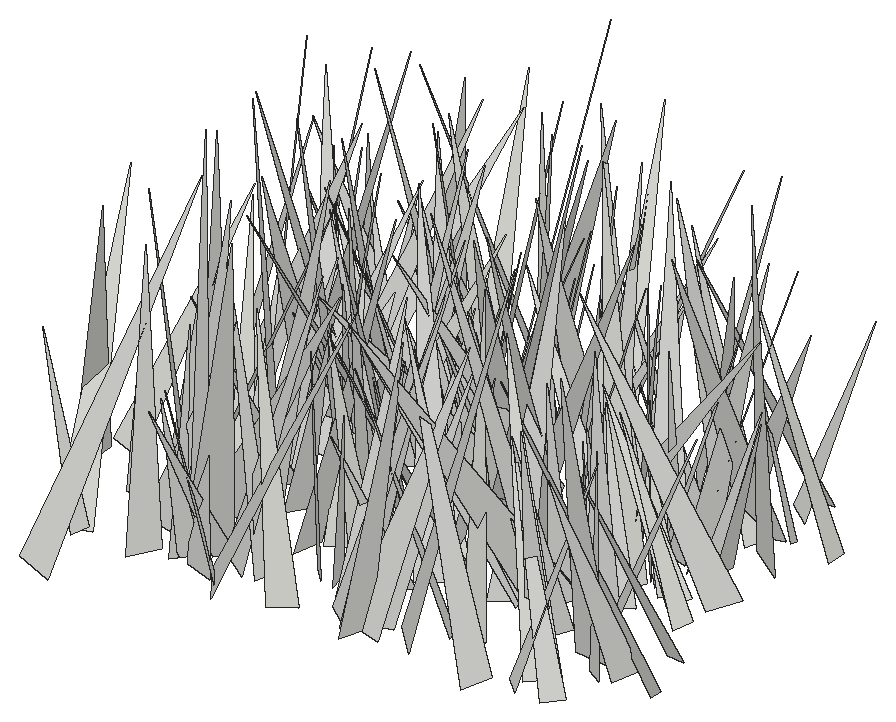
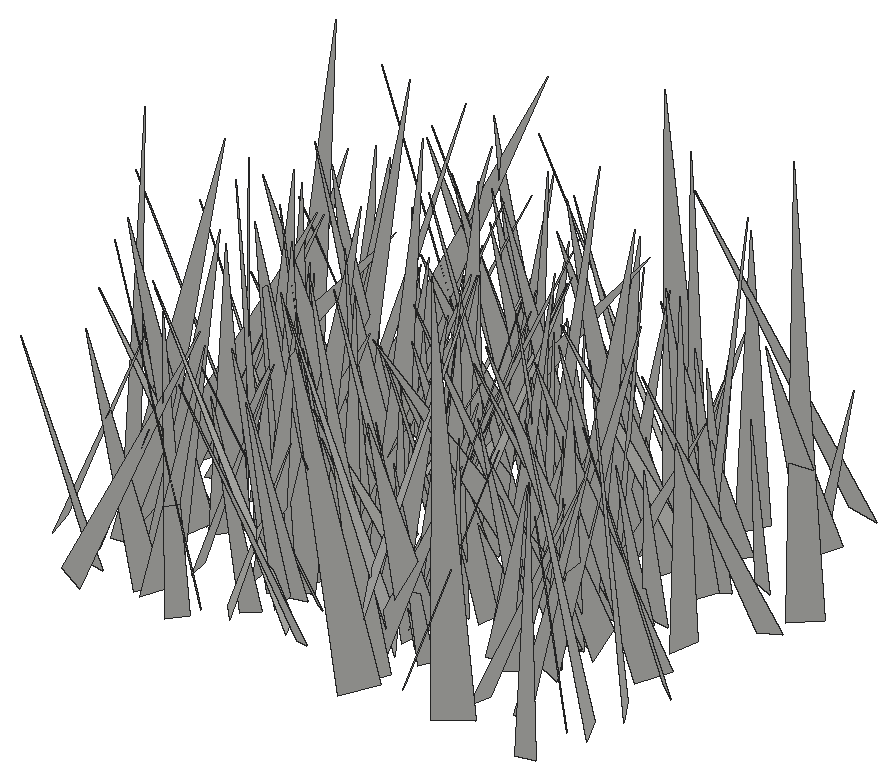
# SketchUp Ruby script. Lengths in inches.
U = 1.inch
M = Sketchup.active_model
def pt(a) = Geom::Point3d.new(a.map { |v| v * U })
def face(e, loops, mat)
  f = e.add_face(loops[0].map { |a| pt(a) })
  loops[1..].each { |l| e.add_face(l.map { |a| pt(a) }).erase! }
  f.material = f.back_material = mat if mat
  f
end
# faces: each face lists its corners as indices into pts; further lists are holes
def faces(e, pts, list, mat = nil) = list.each { |f| face(e, (f[0].is_a?(Array) ? f : [f]).map { |l| l.map { |i| pts[i] } }, mat) }
# xy, xz, yz: faces in a plane at the given z, y or x. An outline is a flat list of corners, or four numbers for a rectangle; further outlines are holes
def ring(l) = l.size == 4 ? [[l[0], l[1]], [l[2], l[1]], [l[2], l[3]], [l[0], l[3]]] : l.each_slice(2).to_a
def flat(e, list, mat, &to3) = list.each { |f| face(e, (f[0].is_a?(Array) ? f : [f]).map { |l| ring(l).map { |u, v| to3.(u, v) } }, mat) }
def xy(e, z, list, mat = nil) = flat(e, list, mat) { |x, y| [x, y, z] }
def xz(e, y, list, mat = nil) = flat(e, list, mat) { |x, z| [x, y, z] }
def yz(e, x, list, mat = nil) = flat(e, list, mat) { |y, z| [x, y, z] }
def lines(e, pts, list) = list.each { |a, b| e.add_line(pt(pts[a]), pt(pts[b])) }
# prism: a flat outline (further loops are holes) pulled along v
def prism(e, loops, v, mat = nil)
  f = face(e, loops, mat); d = Geom::Vector3d.new(v.map { |x| x * U })
  f.pushpull(f.normal.samedirection?(d) ? d.length : -d.length)
end
def box(e, o, s, mat = nil) = prism(e, [[o, [o[0] + s[0], o[1], o[2]], [o[0] + s[0], o[1] + s[1], o[2]], [o[0], o[1] + s[1], o[2]]]], [0, 0, s[2]], mat)
def at(x, y, z, deg = 0) = Geom::Transformation.translation(pt([x, y, z])) * Geom::Transformation.rotation(ORIGIN, Z_AXIS, deg.degrees)
def axes(o, x, y, z) = Geom::Transformation.new([*x, 0, *y, 0, *z, 0, *pt(o).to_a, 1])
def part(name) = M.definitions.add(name)
# library, detail: a bought-in or finely detailed component or shape, given as its bounding box
def library(name, o, s) = part(name).tap { |d| box(d.entities, o, s) }
def detail(e, o, s) = box(e.add_group.entities, o, s)
def put(e, d, t, mat = nil) = e.add_instance(d, t).tap { |i| i.material = mat if mat }
def group(e, t, mat = nil) = e.add_group.tap { |g| g.transformation = t; g.material = mat if mat }.entities
root = M.entities
c1 = part("fur_instance\#9")
p = [[0.8125,0,1.79],[0.67,-0.02,1.48],[0,-0.11,0],[0,0.11,0]]
faces(c1.entities,p,[[0,1,2,3]])
put(root,c1,axes([114.3,322.1,-27.1],[2.50136,7.65725,0.1478],[7.63522,-2.48107,-0.67805],[0.59891,-0.35058,8.02686]))
put(root,c1,axes([118.09,326.15,-27.1],[2.18541,-3.04998,0.78828],[-3.02604,-2.29919,-0.50659],[-0.87571,0.3334,3.71777]))
put(root,c1,axes([118.98,326.99,-27.1],[1.51991,-3.61395,0.26794],[-3.4425,-1.53065,-1.11749],[-1.13207,-0.1975,3.75792]))
put(root,c1,axes([113.92,325.17,-27.1],[-3.79892,0.58903,0.61511],[0.5899,3.84804,-0.04166],[0.61427,-0.05255,3.84409]))
put(root,c1,axes([126.1,325.44,-27.1],[6.14943,-1.42717,1.61929],[-1.52874,-6.3314,0.22535],[-1.52376,0.59247,6.30885]))
put(root,c1,axes([118.09,327.24,-27.1],[6.18232,-5.30847,0.7026],[-5.32058,-6.21081,-0.10875],[-0.60412,0.37485,8.14795]))
put(root,c1,axes([119.89,325.15,-27.1],[5.9079,4.20697,0.32991],[4.15488,-5.69984,-1.72033],[0.73785,-1.5887,7.04573]))
put(root,c1,axes([120.04,325.17,-27.1],[-3.12705,-1.8127,0.50032],[-1.87769,2.95706,-1.02213],[-0.10232,1.13341,3.46693]))
put(root,c1,axes([116.66,325.34,-27.1],[-5.0872,2.66073,2.45988],[2.85923,5.55214,-0.09239],[2.22604,-1.05084,5.74025]))
put(root,c1,axes([122.9,325.35,-27.1],[-2.01026,5.06538,1.49078],[5.275,1.85579,0.80751],[-0.23431,-1.67916,5.38954]))
put(root,c1,axes([131.7,325.32,-27.1],[-6.69944,1.03913,0.45559],[1.00559,6.70154,-0.49804],[0.5255,0.42362,6.76123]))
put(root,c1,axes([125.62,325.96,-27.1],[5.24089,-0.83273,1.62957],[-1.05437,-5.41429,0.62423],[-1.49573,0.89885,5.2698]))
put(root,c1,axes([126.2,325.74,-27.1],[0.11042,6.13884,2.00494],[6.14565,0.51615,-1.91884],[1.98398,-1.94051,5.83229]))
put(root,c1,axes([111.09,329.36,-27.1],[8.00988,-2.00577,0.3429],[-1.833,-7.71682,-2.32157],[-0.88363,-2.17404,7.92412]))
put(root,c1,axes([119.03,325.49,-27.1],[2.99088,7.34321,2.70362],[7.47912,-3.53374,1.32409],[-2.30112,-1.94104,7.81761]))
put(root,c1,axes([134.58,326.01,-27.1],[-1.36293,4.52681,0.55653],[4.38086,1.13777,1.47406],[-1.26877,-0.93423,4.49185]))
put(root,c1,axes([117.8,325.8,-27.1],[-4.10668,0.43412,1.0008],[0.12519,4.05996,-1.24738],[1.0837,1.17608,3.93666]))
put(root,c1,axes([132.625,327.89,-27.1],[1.7038,-4.78318,1.39426],[-4.94528,-1.80274,-0.14134],[-0.60574,1.26373,5.0756]))
put(root,c1,axes([119.65,326.68,-27.1],[3.29943,5.39851,1.49465],[5.593,-3.07886,-1.22601],[0.31023,-1.9081,6.20701]))
put(root,c1,axes([133.89,329.24,-27.1],[0.64901,-7.30772,0.94418],[-7.33385,-0.54888,0.79295],[0.71332,1.00569,7.2935]))
put(root,c1,axes([132.78,325.99,-27.1],[3.07177,3.42083,0.35758],[3.42072,-3.08846,0.16062],[-0.35863,-0.15826,4.59478]))
put(root,c1,axes([135.51,329.01,-27.1],[3.42862,-3.42654,1.21049],[-3.04602,-3.61734,-1.61199],[-1.98197,-0.36822,4.57144]))
put(root,c1,axes([127.79,326.19,-27.1],[5.42391,5.6075,1.42758],[5.74422,-5.4537,-0.40246],[-0.69711,-1.3092,7.79108]))
put(root,c1,axes([115.7,327.26,-27.1],[1.80806,-4.3936,1.6396],[-4.55829,-1.23367,1.72079],[1.10181,2.10605,4.4285]))
put(root,c1,axes([123.3,328.03,-27.1],[3.69206,0.52175,1.19179],[0.74035,-3.79133,-0.63373],[-1.0698,-0.8231,3.6745]))
put(root,c1,axes([128.84,327.54,-27.1],[-4.50374,-2.5863,0.2222],[-2.55985,4.35118,-1.23954],[-0.43072,1.18335,5.04343]))
put(root,c1,axes([130.17,331.65,-27.1],[4.91107,-6.51993,1.1851],[-5.42781,-4.80392,-3.93621],[-3.80168,-1.5638,7.15082]))
put(root,c1,axes([121.08,326.69,-27.1],[-5.72971,0.10944,0.75393],[-0.02545,5.68949,-1.01935],[0.7614,1.01378,5.63937]))
put(root,c1,axes([124.99,325.97,-27.1],[4.48947,6.23838,0.89691],[6.27438,-4.52789,0.08708],[-0.59503,-0.67674,7.68539]))
put(root,c1,axes([115.95,328.92,-27.1],[-4.21383,-5.23135,2.06774],[-5.35043,4.52497,0.54449],[1.7365,1.24763,6.69529]))
put(root,c1,axes([133.375,326.9375,-27.1],[-3.60307,5.2202,0.86904],[5.28801,3.51043,0.83765],[-0.20649,-1.18922,6.28736]))
put(root,c1,axes([125.52,329.08,-27.1],[0.6602,-3.48398,0.63366],[-3.31771,-0.83389,-1.12823],[-1.23791,0.37685,3.36171]))
put(root,c1,axes([113.64,325.14,-27.1],[-5.02723,4.35262,0.08247],[4.19421,4.87628,-1.68986],[1.1665,1.22544,6.43138]))
put(root,c1,axes([122.49,327.96,-27.1],[2.78644,2.89477,1.9564],[3.12581,-3.18339,0.25829],[-1.56092,-1.20736,4.00964]))
put(root,c1,axes([124.03,328.77,-27.1],[2.18387,-4.44969,1.85832],[-4.59717,-2.53702,-0.67228],[-1.45572,1.33648,4.91091]))
put(root,c1,axes([126.52,326.375,-27.1],[-3.94538,2.89092,1.6801],[2.22143,4.20848,-2.02488],[2.49909,0.82308,4.45234]))
put(root,c1,axes([124.66,326.99,-27.1],[0.1573,5.82785,1.1486],[5.93788,-0.12389,-0.18455],[0.15705,-1.15268,5.82705]))
put(root,c1,axes([124.28,327.71,-27.1],[6.01682,-1.89651,1.60783],[-2.22,-5.99358,1.23799],[-1.11958,1.69241,6.18597]))
put(root,c1,axes([134.61,328.35,-27.1],[2.05844,3.54151,1.67651],[3.74882,-2.33096,0.32115],[-1.13989,-1.27062,4.08367]))
put(root,c1,axes([131.76,329.93,-27.1],[3.25434,-3.10316,1.28908],[-2.93626,-3.49873,-1.00964],[-1.63392,0.10675,4.38189]))
put(root,c1,axes([116.9,329.35,-27.1],[3.69144,-5.31541,0.62902],[-5.0613,-3.21782,2.51095],[1.74141,1.9152,5.96452]))
put(root,c1,axes([128.98,331.41,-27.1],[-6.06549,-1.51995,0.44377],[-1.27134,5.72216,2.22212],[0.94386,-2.06007,5.84487]))
put(root,c1,axes([137.13,328.66,-27.1],[-3.79929,-4.93063,0.76728],[-4.2284,2.66909,-3.78564],[-2.64961,2.81057,4.94112]))
put(root,c1,axes([113.76,328.44,-27.1],[0.89714,3.83975,1.01573],[3.88067,-1.06922,0.61438],[-0.84607,-0.83267,3.89501]))
put(root,c1,axes([114.77,329.67,-27.1],[1.60896,-4.17155,1.4473],[-4.41412,-1.4813,0.63763],[0.1098,1.57772,4.42538]))
put(root,c1,axes([129.64,327.76,-27.1],[1.15539,6.15443,1.22459],[6.01284,-1.44203,1.57415],[-1.79512,-0.86897,6.06086]))
put(root,c1,axes([123.45,329.53,-27.1],[2.89079,5.81329,3.19782],[6.3896,-3.37876,0.3661],[-1.787,-2.67707,6.48205]))
put(root,c1,axes([136.08,331.08,-27.1],[-1.33885,-4.31341,0.19295],[-4.24788,1.27969,-0.86785],[-0.77346,0.43835,4.43226]))
put(root,c1,axes([130.73,330.75,-27.1],[-7.92829,-1.68885,1.19775],[-1.65667,8.01779,0.33921],[1.24187,-0.08605,8.09907]))
put(root,c1,axes([127.43,330.625,-27.1],[-4.42248,-6.55022,0.11235],[-5.68971,3.77318,-3.9833],[-3.24733,2.30957,6.8262]))
put(root,c1,axes([120.95,329.23,-27.1],[6.83211,0.09479,1.62922],[-0.11306,-6.96812,0.87954],[-1.62805,0.88169,6.77592]))
put(root,c1,axes([118.62,329.55,-27.1],[6.64236,-2.17739,2.19825],[-2.53423,-6.81539,0.90685],[-1.77512,1.5823,6.93106]))
put(root,c1,axes([122.98,332.32,-27.1],[-2.64137,-6.46023,1.04071],[-6.35863,2.79897,1.23619],[1.54452,0.47506,6.86901]))
put(root,c1,axes([124.71,330.68,-27.1],[-2.99975,-3.60869,1.08185],[-3.74003,3.01886,-0.30041],[0.45307,1.02732,4.68304]))
put(root,c1,axes([125.92,331.4,-27.1],[-2.72161,-4.19987,1.18368],[-4.18397,2.90781,0.69726],[1.23872,0.59401,4.95579]))
put(root,c1,axes([124.97,331.92,-27.1],[-3.4454,-3.89131,0.03074],[-3.88746,3.44363,0.20759],[0.17579,-0.11462,5.19326]))
put(root,c1,axes([115.02,330.32,-27.1],[5.24676,-2.59436,1.90695],[-2.83441,-5.4512,0.38233],[-1.5275,1.20389,5.84064]))
put(root,c1,axes([118.98,331.13,-27.1],[3.98619,-2.41358,0.43201],[-2.42835,-4.00018,0.05811],[-0.33929,0.27366,4.65958]))
put(root,c1,axes([133.05,329.99,-27.1],[-3.3024,-1.44134,1.34219],[-1.74105,3.36144,-0.674],[0.92071,1.18661,3.53964]))
put(root,c1,axes([121.53,331.09,-27.1],[-4.43723,-6.45792,2.6794],[-6.95056,4.4181,-0.86196],[0.75734,2.71083,7.78786]))
put(root,c1,axes([126.05,330.15,-27.1],[-4.29093,5.93832,1.73067],[6.14946,4.32229,0.41585],[0.66564,-1.65078,7.31456]))
put(root,c1,axes([130.49,331.65,-27.1],[3.95695,-1.9726,1.7752],[-1.97238,-4.31833,-0.40205],[-1.77544,0.40099,4.40306]))
put(root,c1,axes([126.03,330.97,-27.1],[3.90442,0.1948,1.09665],[0.0575,-4.02752,0.51071],[-1.11233,0.47558,3.87577]))
put(root,c1,axes([115.68,329.46,-27.1],[5.65943,2.62486,0.30549],[2.50558,-5.55953,1.3513],[-0.8398,1.10185,6.0904]))
put(root,c1,axes([117.69,332.48,-27.1],[-0.92246,-4.02488,0.49642],[-3.83236,0.69867,-1.45667],[-1.32631,0.78053,3.86377]))
put(root,c1,axes([132.05,332.01,-27.1],[4.08918,-3.36848,1.98263],[-3.52303,-4.41912,-0.24183],[-1.69286,1.05996,5.29241]))
put(root,c1,axes([120.55,333.3125,-27.1],[2.722,-4.21365,0.18087],[-4.20663,-2.72794,-0.24377],[-0.30292,0.01939,5.01046]))
put(root,c1,axes([132.64,331.9,-27.1],[4.18709,2.7222,0.51054],[2.74144,-3.94162,-1.4666],[0.39441,-1.502,4.77401]))
put(root,c1,axes([126.26,330.76,-27.1],[-4.785,3.6619,0.62252],[3.69492,4.79647,0.18627],[0.38032,-0.52686,6.02254]))
put(root,c1,axes([128.17,334.47,-27.1],[-1.4202,-8.16889,0.91065],[-8.13373,1.52988,1.03868],[1.18423,0.71114,8.22611]))
put(root,c1,axes([118.68,330.52,-27.1],[-6.74078,-2.87477,2.26806],[-3.46071,6.55422,-1.97791],[1.19661,2.76122,7.05622]))
put(root,c1,axes([125.06,332.03,-27.1],[-5.1041,-1.8904,0.52095],[-1.9461,5.06157,-0.70004],[0.24022,0.83889,5.39772]))
put(root,c1,axes([131.35,333.02,-27.1],[3.43553,-2.13589,0.95207],[-2.02418,-3.56342,-0.68999],[-1.17096,-0.10667,3.98608]))
put(root,c1,axes([121.74,329.93,-27.1],[-4.67511,2.29396,0.21165],[2.12082,4.47274,-1.63107],[0.89953,1.37696,4.94555]))
put(root,c1,axes([128.85,330.68,-27.1],[5.55139,-3.03279,3.66915],[-4.09539,-5.91606,1.30628],[-2.42657,3.04644,6.18946]))
put(root,c1,axes([127.66,333.24,-27.1],[-3.40896,-3.60182,1.17644],[-3.63778,3.55381,0.3393],[1.06005,0.61272,4.94762]))
put(root,c1,axes([111.49,330.83,-27.1],[0.65579,5.75921,0.77226],[5.58682,-0.41126,-1.67728],[1.5976,-0.92592,5.54845]))
put(root,c1,axes([122.79,330.64,-27.1],[3.66563,6.83822,1.35122],[6.90712,-3.76874,0.33492],[-0.93742,-1.02919,7.75151]))
put(root,c1,axes([123.39,337.09,-27.1],[-6.54697,-3.05595,0.68846],[-2.14459,5.53525,4.1758],[2.28332,-3.56338,5.89613]))
put(root,c1,axes([116.68,332.58,-27.1],[2.49544,-4.2024,1.5625],[-4.46283,-2.15679,1.32672],[0.42981,2.0042,4.70396]))
put(root,c1,axes([119.15,333.97,-27.1],[4.7247,0.27251,1.48983],[0.66278,-4.76043,-1.23114],[-1.36183,-1.37139,4.56961]))
put(root,c1,axes([113.26,333.5,-27.1],[6.40054,-0.55178,2.21578],[-0.37829,-6.75939,-0.5905],[-2.25189,-0.43282,6.39709]))
put(root,c1,axes([116.55,335.78,-27.1],[2.6634,-7.09113,0.13913],[-7.08626,-2.66678,-0.26525],[-0.29724,0.03689,7.57017]))
put(root,c1,axes([132.38,332.81,-27.1],[-1.64307,3.38565,0.94063],[3.51296,1.55882,0.52563],[-0.08077,-1.0745,3.72639]))
put(root,c1,axes([134.79,333.09,-27.1],[-3.98782,0.86871,0.11292],[0.87287,3.98492,0.16912],[0.07423,-0.18933,4.07783]))
put(root,c1,axes([125.3,335.3125,-27.1],[4.0127,-3.86264,0.72099],[-3.71726,-4.06564,-1.09277],[-1.27351,-0.30356,5.46147]))
put(root,c1,axes([119.8,334.57,-27.1],[-1.12963,-3.6746,0.26296],[-3.62855,1.06225,-0.74377],[-0.63679,0.46567,3.77168]))
put(root,c1,axes([125.83,337.16,-27.1],[-6.83742,-2.67371,1.15288],[-1.91772,6.34944,3.35188],[2.19094,-2.7864,6.53176]))
put(root,c1,axes([123.98,337.08,-27.1],[7.80685,-2.34529,0.78759],[-1.91376,-7.37702,-2.99744],[-1.56786,-2.67335,7.58041]))
put(root,c1,axes([115.52,332.875,-27.1],[0.0321,3.78164,0.61426],[3.82721,-0.05969,0.16749],[-0.17489,-0.6122,3.77806]))
put(root,c1,axes([129.6,331.84,-27.1],[5.08694,2.79276,1.06084],[2.31416,-5.00849,2.08845],[-1.88933,1.38471,5.41433]))
put(root,c1,axes([122.38,335.94,-27.1],[-4.64993,-4.92524,0.42817],[-4.93518,4.6591,-0.00251],[0.29211,0.31306,6.77347]))
put(root,c1,axes([135.03,335.15,-27.1],[-3.6368,4.97548,2.15784],[5.29036,2.68314,2.72961],[-1.1932,-3.26854,5.52548]))
put(root,c1,axes([133.67,334.3125,-27.1],[-3.19624,2.75407,0.40141],[2.73336,2.9911,1.24258],[-0.52417,-1.19599,4.03198]))
put(root,c1,axes([115.23,332.625,-27.1],[-0.56854,4.75375,0.07359],[4.64609,0.5398,1.02436],[-1.0087,-0.19303,4.67676]))
put(root,c1,axes([131.26,335.68,-27.1],[-4.22534,-4.50008,2.6097],[-4.33201,4.90527,1.44456],[2.88009,0.77613,6.00146]))
put(root,c1,axes([126.45,334.375,-27.1],[6.91635,-1.96319,0.7746],[-2.05636,-6.86586,0.95992],[-0.47486,1.1384,7.12521]))
put(root,c1,axes([125.375,333.96,-27.1],[7.84011,2.17766,1.89393],[2.14429,-8.06482,0.39652],[-1.93163,-0.114,8.12726]))
put(root,c1,axes([126.08,334.66,-27.1],[-4.47703,-2.46915,0.00102],[-2.34184,4.24552,-1.62229],[-0.78262,1.42103,4.84857]))
put(root,c1,axes([117.35,334.88,-27.1],[5.44742,2.57642,1.57153],[2.74581,-5.57692,-0.37485],[-1.25227,-1.0208,6.0143]))
put(root,c1,axes([131.55,333.95,-27.1],[-7.28379,2.71503,1.56111],[2.64145,7.44897,-0.63058],[1.68261,0.05921,7.74773]))
put(root,c1,axes([130.53,335.82,-27.1],[5.81902,2.09502,1.94943],[2.48849,-5.88572,-1.1028],[-1.4131,-1.7377,6.08555]))
put(root,c1,axes([121.86,334.48,-27.1],[0.71871,3.7725,0.80138],[3.83913,-0.62217,-0.51422],[0.36739,-0.87844,3.80576]))
put(root,c1,axes([116.65,333.52,-27.1],[1.55452,5.85258,0.28483],[5.77094,-1.47817,-1.12324],[1.01494,-0.55917,5.95042]))
put(root,c1,axes([124.1,335.99,-27.1],[0.22689,-3.51122,0.97081],[-3.62685,-0.12635,0.39066],[0.3422,0.98893,3.49679]))
put(root,c1,axes([130.54,334.69,-27.1],[-2.56552,5.11443,0.44811],[4.78646,2.20153,2.27666],[-1.85689,-1.39139,5.24939]))
put(root,c1,axes([122.05,335.07,-27.1],[2.7927,4.03544,0.85961],[4.11922,-2.66751,-0.85986],[0.23622,-1.19268,4.83163]))
put(root,c1,axes([118.55,337.15,-27.1],[-2.6676,-6.3456,1.58153],[-6.4273,2.85927,0.63121],[1.20736,1.20081,6.85451]))
put(root,c1,axes([133.08,334.5,-27.1],[-0.96186,4.58475,0.31518],[4.19254,0.74357,1.97843],[-1.88199,-0.68675,4.24628]))
put(root,c1,axes([131.32,332.92,-27.1],[-7.41355,2.38035,1.13819],[1.92535,7.2016,-2.52036],[1.80404,2.09598,7.36713]))
put(root,c1,axes([133.66,335.57,-27.1],[1.6531,3.56586,0.9383],[3.65871,-1.45863,-0.90264],[0.45784,-1.21883,3.82535]))
put(root,c1,axes([119.42,335.28,-27.1],[-0.23432,4.6061,1.3303],[4.44797,-0.2882,1.78136],[-1.78924,-1.31967,4.25416]))
put(root,c1,axes([128.08,337.29,-27.1],[5.88193,4.68919,0.48239],[4.10623,-4.71789,-4.20698],[2.31519,-3.54559,6.23594]))
put(root,c1,axes([122.81,336.21,-27.1],[-3.89073,-0.42692,0.42553],[-0.44504,3.90915,-0.14719],[0.40654,0.19356,3.91132]))
put(root,c1,axes([131.64,336.6875,-27.1],[-0.96334,-4.21277,1.52504],[-4.43315,1.12201,0.29911],[0.64835,1.41239,4.31115]))
put(root,c1,axes([129.72,335.33,-27.1],[-5.3119,3.70536,1.5571],[3.75007,5.49761,-0.28937],[1.44609,-0.64586,6.4701]))
put(root,c1,axes([127.46,335.77,-27.1],[-4.33935,-4.28478,3.74469],[-5.00881,5.11096,0.04388],[2.70071,2.59437,6.09815]))
put(root,c1,axes([132.02,334.92,-27.1],[3.70568,3.40586,0.49894],[3.35111,-3.73706,0.62078],[-0.78668,0.12425,4.99466]))
put(root,c1,axes([115.99,337.87,-27.1],[-2.53564,-6.45433,1.27855],[-6.57975,2.48748,-0.49186],[0.00081,1.3699,6.91708]))
put(root,c1,axes([133.48,337.02,-27.1],[3.83276,-0.80553,0.30542],[-0.78769,-3.84079,-0.24507],[-0.34886,-0.17786,3.90882]))
put(root,c1,axes([118.94,335.74,-27.1],[0.50211,5.33526,1.29674],[5.04367,0.06639,-2.22613],[2.16978,-1.38897,4.87457]))
put(root,c1,axes([112.73,335.83,-27.1],[4.48664,-4.30175,1.96808],[-4.72578,-3.95369,2.13158],[0.21294,2.89338,5.83878]))
put(root,c1,axes([126.22,335.2,-27.1],[-6.64988,-1.58039,2.79885],[-2.32051,6.81074,-1.66765],[2.22405,2.38079,6.62853]))
put(root,c1,axes([126.61,338.82,-27.1],[2.5513,-6.67742,1.15565],[-6.68995,-2.67869,-0.70836],[-1.08074,0.81812,7.11304]))
put(root,c1,axes([133.07,339.86,-27.1],[1.39715,-7.46285,0.32526],[-7.45597,-1.41344,-0.40331],[-0.45656,0.24497,7.58179]))
put(root,c1,axes([119.8125,335.89,-27.1],[-4.5359,3.17744,2.60533],[2.766,5.23085,-1.56386],[3.0386,-0.01843,5.3127]))
put(root,c1,axes([121.87,338.03,-27.1],[-4.72321,-4.87597,2.05821],[-5.0831,4.94763,0.05633],[1.47426,1.43735,6.78828]))
put(root,c1,axes([111.76,336.32,-27.1],[3.62165,4.35293,0.90177],[4.41878,-3.65214,-0.11732],[-0.48531,-0.76904,5.66132]))
put(root,c1,axes([121.12,336.91,-27.1],[-2.98056,5.41129,1.99239],[5.72855,3.03527,0.32601],[0.65987,-1.90801,6.16924]))
put(root,c1,axes([134.3125,338.375,-27.1],[3.79237,5.90894,3.79832],[6.9076,-3.92109,-0.79686],[-1.27587,-3.6653,6.97586]))
put(root,c1,axes([122.59,336.99,-27.1],[-0.71726,5.0627,1.58469],[5.02661,0.13746,1.836],[-1.69568,-1.73401,4.77227]))
put(root,c1,axes([116.52,335.94,-27.1],[2.2285,7.10603,0.93052],[7.02267,-1.97084,-1.76797],[1.42959,-1.39565,7.23438]))
put(root,c1,axes([116.18,336.87,-27.1],[2.91004,3.86675,2.0314],[3.84438,-3.42612,1.0144],[-2.0734,-0.92551,4.73192]))
put(root,c1,axes([126.39,338.23,-27.1],[6.40795,-1.734,1.03011],[-1.73088,-6.48917,-0.15614],[-1.03535,0.11648,6.63658]))
put(root,c1,axes([115.55,335.16,-27.1],[-6.44163,0.17845,3.84936],[-1.24896,6.99677,-2.4144],[3.64548,2.71245,5.9747]))
put(root,c1,axes([116.66,335.99,-27.1],[-2.09458,6.39775,0.76013],[6.40195,1.97698,1.00139],[-0.72385,-1.02792,6.657]))
put(root,c1,axes([122.02,337.7,-27.1],[-7.0839,-2.86843,1.00142],[-2.98784,7.03787,-0.97651],[0.55097,1.28563,7.57997]))
put(root,c1,axes([116.6875,334.89,-27.1],[-2.61013,7.00123,1.33294],[6.01827,2.92557,-3.58165],[3.81765,0.17478,6.55758]))
put(root,c1,axes([131.94,337.63,-27.1],[5.79665,-1.91222,1.6292],[-2.17494,-5.87047,0.84811],[-1.25719,1.33905,6.04471]))
put(root,c1,axes([116.87,337.66,-27.1],[0.82444,4.69785,1.50621],[4.90559,-0.61872,-0.75536],[0.52313,-1.60174,4.70945]))
put(root,c1,axes([130.95,337.02,-27.1],[-5.28353,4.19242,1.51467],[4.2139,5.46353,-0.42331],[1.45386,-0.59977,6.73148]))
put(root,c1,axes([122.89,338.15,-27.1],[-6.49588,1.72746,1.45223],[1.82521,6.62397,0.28488],[1.32729,-0.65455,6.71561]))
put(root,c1,axes([124.64,336.65,-27.1],[3.32895,2.2471,0.95718],[1.81279,-3.35751,1.57751],[-1.63691,0.85163,3.69362]))
put(root,c1,axes([125.71,336.78,-27.1],[1.80048,6.74236,1.9451],[6.61582,-2.30046,1.85022],[-2.33959,-1.31645,6.72888]))
put(root,c1,axes([122.62,336.43,-27.1],[4.4552,2.25801,0.37031],[2.04407,-4.29173,1.57715],[-1.02836,1.2518,4.7392]))
put(root,c1,axes([111.95,338.4,-27.1],[5.69134,3.55142,2.30083],[3.82093,-5.97012,-0.23634],[-1.81848,-1.42926,6.70433]))
put(root,c1,axes([132.38,336.43,-27.1],[4.78963,3.34115,0.62659],[3.09789,-4.73577,1.57225],[-1.39963,0.95165,5.62422]))
put(root,c1,axes([123.64,339.4,-27.1],[4.61843,1.91697,0.98697],[2.11588,-4.47821,-1.2031],[-0.41467,-1.49987,4.85358]))
put(root,c1,axes([117.01,338.67,-27.1],[-3.73085,2.02538,0.45172],[2.07172,3.68874,0.57157],[0.11914,-0.71871,4.20651]))
put(root,c1,axes([117.73,338.36,-27.1],[-1.66438,3.94539,0.96796],[4.04045,1.49913,0.83702],[-0.42169,-1.20819,4.19948]))
put(root,c1,axes([120.79,339.13,-27.1],[3.65523,2.01923,0.98653],[2.16689,-3.66612,-0.52479],[-0.59594,-0.94526,4.14277]))
put(root,c1,axes([121.82,337.69,-27.1],[6.24718,3.3719,1.68528],[3.2403,-6.4703,0.93425],[-1.92623,0.05148,7.03734]))
put(root,c1,axes([114.52,341.07,-27.1],[-1.82022,-4.66244,0.24993],[-4.60062,1.83672,0.75812],[0.79693,-0.04591,4.9474]))
put(root,c1,axes([130.1875,339.75,-27.1],[-4.58656,-0.99691,0.53395],[-0.9871,4.61746,0.14195],[0.55187,-0.02624,4.69151]))
put(root,c1,axes([119.61,340.11,-27.1],[3.62629,-0.3933,0.08931],[-0.3696,-3.56406,-0.68808],[-0.16141,-0.67481,3.58206]))
put(root,c1,axes([133.125,339.32,-27.1],[-3.66432,1.46778,0.50332],[1.5223,3.65057,0.437],[0.30055,-0.59495,3.9231]))
put(root,c1,axes([131.15,340.53,-27.1],[1.6386,-6.2759,2.07036],[-6.47654,-1.94928,-0.78297],[-1.31443,1.78093,6.43885]))
put(root,c1,axes([125.04,339.27,-27.1],[3.37481,3.69249,0.11879],[3.55193,-3.19874,-1.47981],[1.01606,-1.08238,4.77849]))
put(root,c1,axes([121.48,340.69,-27.1],[-0.67131,-4.1889,0.93111],[-4.10147,0.34927,-1.38579],[-1.26165,1.09345,4.00962]))
put(root,c1,axes([119.22,341.77,-27.1],[-4.05728,-2.523,0.42943],[-2.40041,4.03064,1.00168],[0.88766,-0.63233,4.67158]))
put(root,c1,axes([128.2,338.3,-27.1],[-7.28792,0.99409,0.70676],[0.80322,7.1337,-1.75122],[0.9179,1.65037,7.1439]))
put(root,c1,axes([121.63,342.37,-27.1],[-5.81753,-5.50464,0.89808],[-5.45533,5.88597,0.73893],[1.16061,0.07452,7.97488]))
put(root,c1,axes([124.1,337.8125,-27.1],[3.59429,3.23742,0.8797],[2.57384,-3.488,2.32011],[-2.15177,1.23558,4.24464]))
put(root,c1,axes([117.62,341.18,-27.1],[4.3427,-1.50818,1.19732],[-1.3579,-4.49272,-0.73402],[-1.36538,-0.32877,4.53816]))
put(root,c1,axes([116.46,341.01,-27.1],[-5.398,0.07669,0.31538],[0.11355,5.36878,0.63804],[0.30406,-0.64352,5.36071]))
put(root,c1,axes([120.31,342.01,-27.1],[7.393,0.04175,0.28729],[0.1077,-7.1937,-1.72622],[-0.26959,-1.72907,7.18877]))
put(root,c1,axes([135.98,340.28,-27.1],[-5.12979,-1.0122,0.11272],[-1.018,5.07872,-0.72273],[-0.03042,0.73083,5.17851]))
put(root,c1,axes([116.33,342.67,-27.1],[2.3597,-7.64104,0.82634],[-7.58316,-2.17409,1.55097],[1.25061,1.23463,7.84527]))
put(root,c1,axes([112.96,340.53,-27.1],[3.09566,2.75124,1.27433],[2.88928,-3.22895,-0.04754],[-0.91941,-0.88367,4.14127]))
put(root,c1,axes([112.03,340.25,-27.1],[5.547,2.87669,1.51326],[2.93945,-5.71712,0.09337],[-1.38744,-0.61131,6.24786]))
put(root,c1,axes([126.76,341.05,-27.1],[-0.37702,3.57753,2.02822],[3.88687,0.97529,-0.99777],[1.34335,-1.81786,3.4562]))
put(root,c1,axes([134.09,340.22,-27.1],[-3.59352,-1.36236,0.30323],[-1.35819,3.22059,-1.62619],[-0.32136,1.6227,3.48208]))
put(root,c1,axes([127.36,341.55,-27.1],[-2.83398,-2.56318,0.53676],[-2.6174,2.79801,-0.45803],[0.08496,0.70049,3.79362]))
put(root,c1,axes([130.67,341.93,-27.1],[3.4493,-3.36014,0.02886],[-3.29462,-3.37365,0.97621],[0.66096,0.719,4.71542]))
put(root,c1,axes([128.57,342.95,-27.1],[5.40312,-1.02873,0.51523],[-0.87968,-5.28821,-1.33359],[-0.74156,-1.2223,5.33606]))
put(root,c1,axes([126.33,339.54,-27.1],[-5.21181,1.32812,1.31914],[0.83689,5.14396,-1.87252],[1.67442,1.56295,5.04188]))
put(root,c1,axes([121.09,338.52,-27.1],[-5.92228,3.52878,0.304],[3.26745,5.67188,-2.1844],[1.36692,1.73077,6.53866]))
put(root,c1,axes([125.08,340.99,-27.1],[6.15209,3.35933,0.33959],[3.37614,-6.1107,-0.71393],[0.04606,-0.78923,6.97306]))
put(root,c1,axes([133.24,343.125,-27.1],[-1.88046,-5.21634,0.33238],[-5.10911,1.75978,-1.28722],[-1.10347,0.74146,5.39346]))
put(root,c1,axes([128.65,341.6,-27.1],[5.36031,4.39922,1.5205],[4.6383,-5.24227,-1.18439],[-0.38885,-1.88772,6.83252]))
put(root,c1,axes([130.35,342.09,-27.1],[-5.09295,0.86723,1.4086],[1.03106,5.23004,0.50795],[1.29351,-0.75432,5.14123]))
put(root,c1,axes([121.52,339.38,-27.1],[6.37842,4.90538,1.53696],[4.59516,-6.53882,1.79932],[-2.30422,0.53885,7.84279]))
put(root,c1,axes([126.4375,339.4,-27.1],[-1.83957,6.80237,0.25254],[6.80704,1.83779,0.08208],[-0.01336,-0.2652,7.04624]))
put(root,c1,axes([112.64,343.1875,-27.1],[-0.50328,-4.91347,1.0032],[-4.85841,0.72759,1.12622],[1.24277,0.85458,4.80907]))
put(root,c1,axes([120.26,343.04,-27.1],[6.42408,-3.63909,0.41323],[-3.66082,-6.40525,0.50369],[-0.11006,0.64215,7.36601]))
put(root,c1,axes([123.97,341.65,-27.1],[2.98745,4.37857,0.43851],[4.21633,-2.69647,-1.80015],[1.25963,-1.35874,4.98559]))
put(root,c1,axes([133,341.94,-27.1],[2.35379,3.88662,0.95748],[3.9563,-2.09005,-1.24191],[0.60851,-1.44527,4.3708]))
